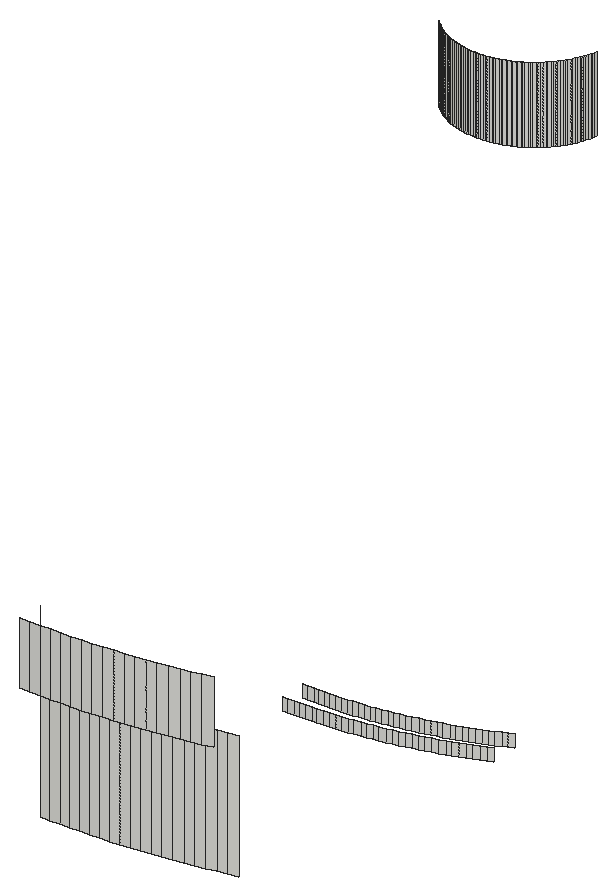
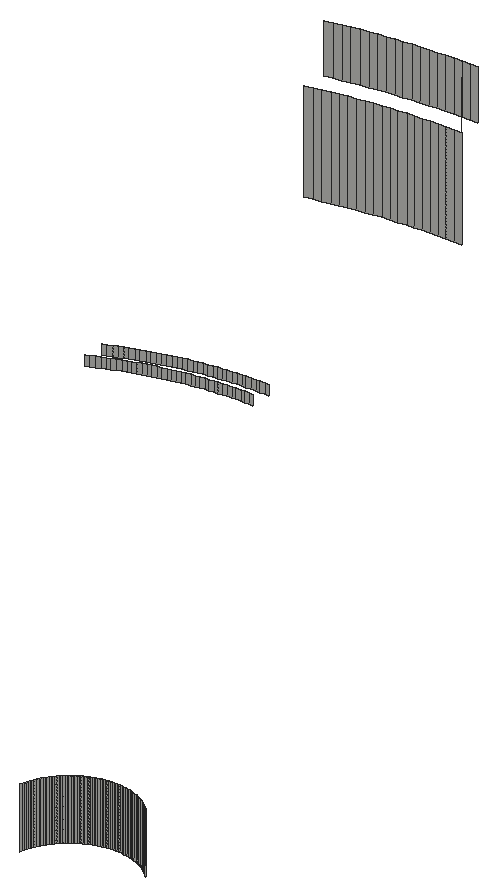
# SketchUp Ruby script. Lengths in inches.
U = 1.inch
M = Sketchup.active_model
def pt(a) = Geom::Point3d.new(a.map { |v| v * U })
def face(e, loops, mat)
  f = e.add_face(loops[0].map { |a| pt(a) })
  loops[1..].each { |l| e.add_face(l.map { |a| pt(a) }).erase! }
  f.material = f.back_material = mat if mat
  f
end
# faces: each face lists its corners as indices into pts; further lists are holes
def faces(e, pts, list, mat = nil) = list.each { |f| face(e, (f[0].is_a?(Array) ? f : [f]).map { |l| l.map { |i| pts[i] } }, mat) }
# xy, xz, yz: faces in a plane at the given z, y or x. An outline is a flat list of corners, or four numbers for a rectangle; further outlines are holes
def ring(l) = l.size == 4 ? [[l[0], l[1]], [l[2], l[1]], [l[2], l[3]], [l[0], l[3]]] : l.each_slice(2).to_a
def flat(e, list, mat, &to3) = list.each { |f| face(e, (f[0].is_a?(Array) ? f : [f]).map { |l| ring(l).map { |u, v| to3.(u, v) } }, mat) }
def xy(e, z, list, mat = nil) = flat(e, list, mat) { |x, y| [x, y, z] }
def xz(e, y, list, mat = nil) = flat(e, list, mat) { |x, z| [x, y, z] }
def yz(e, x, list, mat = nil) = flat(e, list, mat) { |y, z| [x, y, z] }
def lines(e, pts, list) = list.each { |a, b| e.add_line(pt(pts[a]), pt(pts[b])) }
# prism: a flat outline (further loops are holes) pulled along v
def prism(e, loops, v, mat = nil)
  f = face(e, loops, mat); d = Geom::Vector3d.new(v.map { |x| x * U })
  f.pushpull(f.normal.samedirection?(d) ? d.length : -d.length)
end
def box(e, o, s, mat = nil) = prism(e, [[o, [o[0] + s[0], o[1], o[2]], [o[0] + s[0], o[1] + s[1], o[2]], [o[0], o[1] + s[1], o[2]]]], [0, 0, s[2]], mat)
def at(x, y, z, deg = 0) = Geom::Transformation.translation(pt([x, y, z])) * Geom::Transformation.rotation(ORIGIN, Z_AXIS, deg.degrees)
def axes(o, x, y, z) = Geom::Transformation.new([*x, 0, *y, 0, *z, 0, *pt(o).to_a, 1])
def part(name) = M.definitions.add(name)
# library, detail: a bought-in or finely detailed component or shape, given as its bounding box
def library(name, o, s) = part(name).tap { |d| box(d.entities, o, s) }
def detail(e, o, s) = box(e.add_group.entities, o, s)
def put(e, d, t, mat = nil) = e.add_instance(d, t).tap { |i| i.material = mat if mat }
def group(e, t, mat = nil) = e.add_group.tap { |g| g.transformation = t; g.material = mat if mat }.entities
root = M.entities
xz(root,204,[[270,354.5,270.39,357]])
xz(root,205,[[270,349.5,270.38,354.5]])
xz(root,217,[[270,348,270.22,348.5]])
xz(root,217.01,[[270.45,348,270.67,348.5]])
xz(root,218,[[270,348,270.21,348.5]])
xz(root,218.01,[[270.42,348,270.63,348.5]])
xz(root,249,[[251.84,348,251.92,351],[251.92,348,252,351],[252,348,252.08,351],[252.08,348,252.16,351]])
p = [[270.45,217.01,348],[270.22,217,348],[270.22,217,348.5],[270.45,217.01,348.5],[270.89,217.02,348],[270.67,217.01,348],
  [270.67,217.01,348.5],[270.89,217.02,348.5],[271.11,217.04,348],[271.11,217.04,348.5],[271.33,217.05,348],[271.33,217.05,348.5],
  [271.56,217.07,348],[271.56,217.07,348.5],[271.78,217.09,348],[271.78,217.09,348.5],[272,217.12,348],[272,217.12,348.5],
  [272.22,217.15,348],[272.22,217.15,348.5],[272.4375,217.18,348],[272.4375,217.18,348.5],[272.66,217.21,348],[272.66,217.21,348.5],
  [272.88,217.25,348],[272.88,217.25,348.5],[273.1,217.28,348],[273.1,217.28,348.5],[273.32,217.33,348],[273.32,217.33,348.5],
  [273.53,217.37,348],[273.53,217.37,348.5],[273.75,217.42,348],[273.75,217.42,348.5],[273.97,217.47,348],[273.97,217.47,348.5],
  [274.18,217.52,348],[274.18,217.52,348.5],[274.4,217.58,348],[274.4,217.58,348.5],[274.61,217.64,348],[274.61,217.64,348.5],
  [274.83,217.7,348],[274.83,217.7,348.5],[275.04,217.76,348],[275.04,217.76,348.5],[275.25,217.83,348],[275.25,217.83,348.5],
  [275.46,217.9,348],[275.46,217.9,348.5],[275.67,217.98,348],[275.67,217.98,348.5],[270.21,218,348],[270.42,218.01,348],
  [270.42,218.01,348.5],[270.21,218,348.5],[270.63,218.01,348],[270.84,218.02,348],[270.84,218.02,348.5],[270.63,218.01,348.5],
  [271.05,218.03,348],[271.05,218.03,348.5],[271.26,218.05,348],[271.26,218.05,348.5],[271.46,218.07,348],[271.46,218.07,348.5],
  [275.88,218.05,348],[275.88,218.05,348.5],[271.67,218.09,348],[271.67,218.09,348.5],[271.88,218.11,348],[271.88,218.11,348.5],
  [272.09,218.14,348],[272.09,218.14,348.5],[272.3,218.17,348],[272.3,218.17,348.5],[276.09,218.13,348],[276.09,218.13,348.5],
  [276.3,218.21,348],[276.3,218.21,348.5],[272.5,218.2,348],[272.5,218.2,348.5],[272.71,218.23,348],[272.71,218.23,348.5],
  [272.92,218.27,348],[272.92,218.27,348.5],[276.51,218.29,348],[276.51,218.29,348.5],[273.12,218.31,348],[273.12,218.31,348.5],
  [273.33,218.35,348],[273.33,218.35,348.5],[273.53,218.39,348],[273.53,218.39,348.5],[276.71,218.38,348],[276.71,218.38,348.5],
  [273.74,218.44,348],[273.74,218.44,348.5],[273.9375,218.49,348],[273.9375,218.49,348.5],[276.91,218.47,348],[276.91,218.47,348.5],
  [274.14,218.55,348],[274.14,218.55,348.5],[274.34,218.6,348],[274.34,218.6,348.5],[277.12,218.5625,348],[277.12,218.5625,348.5],
  [274.54,218.66,348],[274.54,218.66,348.5],[274.74,218.72,348],[274.74,218.72,348.5],[274.94,218.78,348],[274.94,218.78,348.5],
  [275.14,218.85,348],[275.14,218.85,348.5],[275.34,218.92,348],[275.34,218.92,348.5],[275.54,218.99,348],[275.54,218.99,348.5],
  [275.73,219.0625,348],[275.73,219.0625,348.5],[275.93,219.14,348],[275.93,219.14,348.5],[276.12,219.22,348],[276.12,219.22,348.5],
  [276.32,219.3,348],[276.32,219.3,348.5],[276.51,219.38,348],[276.51,219.38,348.5],[276.7,219.47,348],[276.7,219.47,348.5],
  [276.89,219.56,348],[276.89,219.56,348.5],[277.08,219.65,348],[277.08,219.65,348.5],[251.53,249.04,348],[251.45,249.05,348],
  [251.45,249.05,351],[251.53,249.04,351],[251.61,249.03,348],[251.61,249.03,351],[251.6875,249.02,348],[251.6875,249.02,351],
  [251.76,249.01,348],[251.76,249.01,351],[251.84,249,348],[251.84,249,351],[252.24,249.01,348],[252.16,249,348],
  [252.16,249,351],[252.24,249.01,351],[252.3125,249.02,348],[252.3125,249.02,351],[252.39,249.03,348],[252.39,249.03,351],
  [252.47,249.04,348],[252.47,249.04,351],[252.55,249.05,348],[252.55,249.05,351],[251.07,249.15,348],[251,249.17,348],
  [251,249.17,351],[251.07,249.15,351],[251.15,249.125,348],[251.15,249.125,351],[251.22,249.1,348],[251.22,249.1,351],
  [251.3,249.08,348],[251.3,249.08,351],[251.375,249.07,348],[251.375,249.07,351],[252.625,249.07,348],[252.625,249.07,351],
  [252.7,249.08,348],[252.7,249.08,351],[252.78,249.1,348],[252.78,249.1,351],[252.85,249.125,348],[252.85,249.125,351],
  [252.93,249.15,348],[252.93,249.15,351],[253,249.17,348],[253,249.17,351],[250.85,249.23,348],[250.78,249.26,348],
  [250.78,249.26,351],[250.85,249.23,351],[250.92,249.2,348],[250.92,249.2,351],[253.07,249.2,348],[253.07,249.2,351],
  [253.15,249.23,348],[253.15,249.23,351],[253.22,249.26,348],[253.22,249.26,351],[250.64,249.33,348],[250.57,249.36,348],
  [250.57,249.36,351],[250.64,249.33,351],[250.71,249.29,348],[250.71,249.29,351],[253.29,249.29,348],[253.29,249.29,351],
  [253.36,249.33,348],[253.36,249.33,351],[253.43,249.36,348],[253.43,249.36,351],[250.43,249.44,348],[250.37,249.48,348],
  [250.37,249.48,351],[250.43,249.44,351],[250.5,249.4,348],[250.5,249.4,351],[253.5,249.4,348],[253.5,249.4,351],
  [253.57,249.44,348],[253.57,249.44,351],[253.63,249.48,348],[253.63,249.48,351],[250.3,249.53,348],[250.24,249.57,348],
  [250.24,249.57,351],[250.3,249.53,351],[253.7,249.53,348],[253.7,249.53,351],[253.76,249.57,348],[253.76,249.57,351],
  [250.17,249.62,348],[250.11,249.67,348],[250.11,249.67,351],[250.17,249.62,351],[253.83,249.62,348],[253.83,249.62,351],
  [253.89,249.67,348],[253.89,249.67,351],[250.05,249.72,348],[249.99,249.77,348],[249.99,249.77,351],[250.05,249.72,351],
  [253.95,249.72,348],[253.95,249.72,351],[254.01,249.77,348],[254.01,249.77,351],[249.93,249.82,348],[249.88,249.88,348],
  [249.88,249.88,351],[249.93,249.82,351],[254.06,249.82,348],[254.06,249.82,351],[254.12,249.88,348],[254.12,249.88,351],
  [254.18,249.93,348],[254.18,249.93,351],[254.23,249.99,348],[254.23,249.99,351],[254.28,250.05,348],[254.28,250.05,351],
  [254.33,250.11,348],[254.33,250.11,351],[254.38,250.17,348],[254.38,250.17,351],[254.43,250.24,348],[254.43,250.24,351],
  [254.47,250.3,348],[254.47,250.3,351],[254.52,250.37,348],[254.52,250.37,351],[254.56,250.43,348],[254.56,250.43,351],
  [254.6,250.5,348],[254.6,250.5,351],[254.64,250.57,348],[254.64,250.57,351],[254.67,250.64,348],[254.67,250.64,351],
  [254.71,250.71,348],[254.71,250.71,351],[254.74,250.78,348],[254.74,250.78,351],[254.77,250.85,348],[254.77,250.85,351],
  [254.8,250.92,348],[254.8,250.92,351],[254.83,251,348],[254.83,251,351],[254.85,251.07,348],[254.85,251.07,351],
  [254.875,251.15,348],[254.875,251.15,351],[254.9,251.22,348],[254.9,251.22,351],[254.92,251.3,348],[254.92,251.3,351],
  [254.93,251.375,348],[254.93,251.375,351],[270.38,205,349.5],[270.76,205.01,349.5],[270.76,205.01,354.5],[270.38,205,354.5],
  [271.14,205.02,349.5],[271.14,205.02,354.5],[271.52,205.04,349.5],[271.52,205.04,354.5],[271.9,205.0625,349.5],[271.9,205.0625,354.5],
  [272.28,205.09,349.5],[272.28,205.09,354.5],[272.65,205.12,349.5],[272.65,205.12,354.5],[273.03,205.16,349.5],[273.03,205.16,354.5],
  [273.41,205.2,349.5],[273.41,205.2,354.5],[273.79,205.25,349.5],[273.79,205.25,354.5],[274.16,205.3,349.5],[274.16,205.3,354.5],
  [274.54,205.36,349.5],[274.54,205.36,354.5],[274.91,205.42,349.5],[274.91,205.42,354.5],[275.28,205.49,349.5],[275.28,205.49,354.5],
  [275.66,205.56,349.5],[275.66,205.56,354.5],[276.03,205.63,349.5],[276.03,205.63,354.5],[276.4,205.72,349.5],[276.4,205.72,354.5],
  [276.77,205.8,349.5],[276.77,205.8,354.5],[277.14,205.89,349.5],[277.14,205.89,354.5],[270.39,204,354.5],[270.79,204.01,354.5],
  [270.79,204.01,357],[270.39,204,357],[271.18,204.02,354.5],[271.18,204.02,357],[271.57,204.04,354.5],[271.57,204.04,357],
  [271.96,204.0625,354.5],[271.96,204.0625,357],[272.35,204.09,354.5],[272.35,204.09,357],[272.75,204.125,354.5],[272.75,204.125,357],
  [273.14,204.16,354.5],[273.14,204.16,357],[273.53,204.21,354.5],[273.53,204.21,357],[273.92,204.26,354.5],[273.92,204.26,357],
  [274.3,204.31,354.5],[274.3,204.31,357],[274.69,204.37,354.5],[274.69,204.37,357],[275.08,204.43,354.5],[275.08,204.43,357],
  [275.47,204.5,354.5],[275.47,204.5,357],[275.85,204.58,354.5],[275.85,204.58,357],[276.24,204.66,354.5],[276.24,204.66,357],
  [276.62,204.74,354.5],[276.62,204.74,357],[277,204.83,354.5],[277,204.83,357],[270,205,354.5],[270,205,357]]
faces(root,p,[[0,1,2,3],[4,5,6,7],[8,4,7,9],[10,8,9,11],[12,10,11,13],[14,12,13,15],[16,14,15,17],[18,16,17,19],
  [20,18,19,21],[22,20,21,23],[24,22,23,25],[26,24,25,27],[28,26,27,29],[30,28,29,31],[32,30,31,33],[34,32,33,35],
  [36,34,35,37],[38,36,37,39],[40,38,39,41],[42,40,41,43],[44,42,43,45],[46,44,45,47],[48,46,47,49],[50,48,49,51],
  [52,53,54,55],[56,57,58,59],[57,60,61,58],[60,62,63,61],[62,64,65,63],[66,50,51,67],[64,68,69,65],[68,70,71,69],
  [70,72,73,71],[72,74,75,73],[76,66,67,77],[78,76,77,79],[74,80,81,75],[80,82,83,81],[82,84,85,83],[86,78,79,87],
  [84,88,89,85],[88,90,91,89],[90,92,93,91],[94,86,87,95],[92,96,97,93],[96,98,99,97],[100,94,95,101],[98,102,103,99],
  [102,104,105,103],[106,100,101,107],[104,108,109,105],[108,110,111,109],[110,112,113,111],[112,114,115,113],[114,116,117,115],[116,118,119,117],
  [118,120,121,119],[120,122,123,121],[122,124,125,123],[124,126,127,125],[126,128,129,127],[128,130,131,129],[130,132,133,131],[132,134,135,133],
  [136,137,138,139],[140,136,139,141],[142,140,141,143],[144,142,143,145],[146,144,145,147],[148,149,150,151],[152,148,151,153],[154,152,153,155],
  [156,154,155,157],[158,156,157,159],[160,161,162,163],[164,160,163,165],[166,164,165,167],[168,166,167,169],[170,168,169,171],[137,170,171,138],
  [172,158,159,173],[174,172,173,175],[176,174,175,177],[178,176,177,179],[180,178,179,181],[182,180,181,183],[184,185,186,187],[188,184,187,189],
  [161,188,189,162],[190,182,183,191],[192,190,191,193],[194,192,193,195],[196,197,198,199],[200,196,199,201],[185,200,201,186],[202,194,195,203],
  [204,202,203,205],[206,204,205,207],[208,209,210,211],[212,208,211,213],[197,212,213,198],[214,206,207,215],[216,214,215,217],[218,216,217,219],
  [220,221,222,223],[209,220,223,210],[224,218,219,225],[226,224,225,227],[228,229,230,231],[221,228,231,222],[232,226,227,233],[234,232,233,235],
  [236,237,238,239],[229,236,239,230],[240,234,235,241],[242,240,241,243],[244,245,246,247],[237,244,247,238],[248,242,243,249],[250,248,249,251],
  [252,250,251,253],[254,252,253,255],[256,254,255,257],[258,256,257,259],[260,258,259,261],[262,260,261,263],[264,262,263,265],[266,264,265,267],
  [268,266,267,269],[270,268,269,271],[272,270,271,273],[274,272,273,275],[276,274,275,277],[278,276,277,279],[280,278,279,281],[282,280,281,283],
  [284,282,283,285],[286,284,285,287],[288,286,287,289],[290,288,289,291],[292,290,291,293],[294,292,293,295],[296,297,298,299],[297,300,301,298],
  [300,302,303,301],[302,304,305,303],[304,306,307,305],[306,308,309,307],[308,310,311,309],[310,312,313,311],[312,314,315,313],[314,316,317,315],
  [316,318,319,317],[318,320,321,319],[320,322,323,321],[322,324,325,323],[324,326,327,325],[326,328,329,327],[328,330,331,329],[330,332,333,331],
  [334,335,336,337],[335,338,339,336],[338,340,341,339],[340,342,343,341],[342,344,345,343],[344,346,347,345],[346,348,349,347],[348,350,351,349],
  [350,352,353,351],[352,354,355,353],[354,356,357,355],[356,358,359,357],[358,360,361,359],[360,362,363,361],[362,364,365,363],[364,366,367,365],
  [366,368,369,367]])
lines(root,p,[[370,371]])
